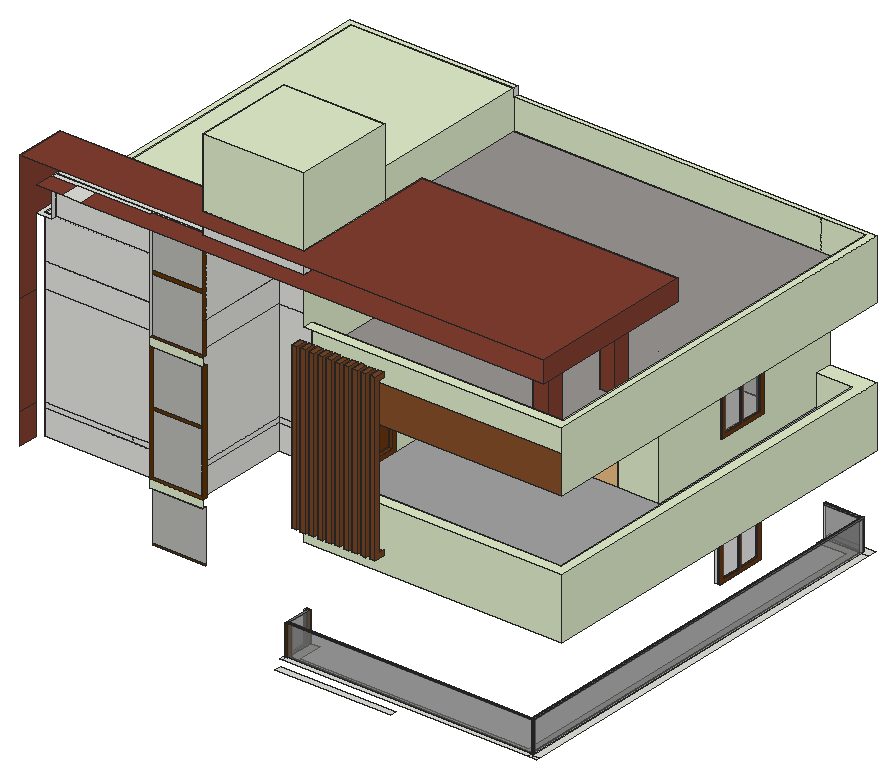
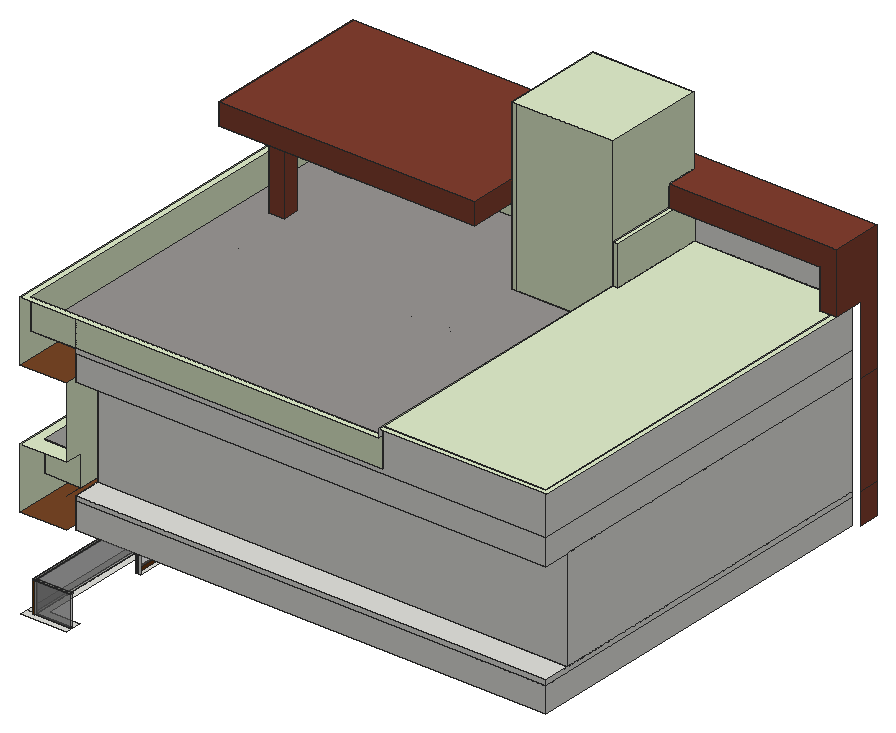
# SketchUp Ruby script. Lengths in inches.
U = 1.inch
M = Sketchup.active_model
def pt(a) = Geom::Point3d.new(a.map { |v| v * U })
def face(e, loops, mat)
  f = e.add_face(loops[0].map { |a| pt(a) })
  loops[1..].each { |l| e.add_face(l.map { |a| pt(a) }).erase! }
  f.material = f.back_material = mat if mat
  f
end
# faces: each face lists its corners as indices into pts; further lists are holes
def faces(e, pts, list, mat = nil) = list.each { |f| face(e, (f[0].is_a?(Array) ? f : [f]).map { |l| l.map { |i| pts[i] } }, mat) }
# xy, xz, yz: faces in a plane at the given z, y or x. An outline is a flat list of corners, or four numbers for a rectangle; further outlines are holes
def ring(l) = l.size == 4 ? [[l[0], l[1]], [l[2], l[1]], [l[2], l[3]], [l[0], l[3]]] : l.each_slice(2).to_a
def flat(e, list, mat, &to3) = list.each { |f| face(e, (f[0].is_a?(Array) ? f : [f]).map { |l| ring(l).map { |u, v| to3.(u, v) } }, mat) }
def xy(e, z, list, mat = nil) = flat(e, list, mat) { |x, y| [x, y, z] }
def xz(e, y, list, mat = nil) = flat(e, list, mat) { |x, z| [x, y, z] }
def yz(e, x, list, mat = nil) = flat(e, list, mat) { |y, z| [x, y, z] }
def lines(e, pts, list) = list.each { |a, b| e.add_line(pt(pts[a]), pt(pts[b])) }
# prism: a flat outline (further loops are holes) pulled along v
def prism(e, loops, v, mat = nil)
  f = face(e, loops, mat); d = Geom::Vector3d.new(v.map { |x| x * U })
  f.pushpull(f.normal.samedirection?(d) ? d.length : -d.length)
end
def box(e, o, s, mat = nil) = prism(e, [[o, [o[0] + s[0], o[1], o[2]], [o[0] + s[0], o[1] + s[1], o[2]], [o[0], o[1] + s[1], o[2]]]], [0, 0, s[2]], mat)
def at(x, y, z, deg = 0) = Geom::Transformation.translation(pt([x, y, z])) * Geom::Transformation.rotation(ORIGIN, Z_AXIS, deg.degrees)
def axes(o, x, y, z) = Geom::Transformation.new([*x, 0, *y, 0, *z, 0, *pt(o).to_a, 1])
def part(name) = M.definitions.add(name)
# library, detail: a bought-in or finely detailed component or shape, given as its bounding box
def library(name, o, s) = part(name).tap { |d| box(d.entities, o, s) }
def detail(e, o, s) = box(e.add_group.entities, o, s)
def put(e, d, t, mat = nil) = e.add_instance(d, t).tap { |i| i.material = mat if mat }
def group(e, t, mat = nil) = e.add_group.tap { |g| g.transformation = t; g.material = mat if mat }.entities
root = M.entities
M.materials.add("[Color A08]").color = [102, 52, 0]
M.materials.add("[Color C08]").color = [82, 45, 0]
M.materials.add("[Concrete Aggregate Smoke]").color = [154, 150, 148]
M.materials.add("[Metal Seamed]").color = [118, 119, 115]
M.materials.add("[Mirror 01]").color = [185, 185, 181]
M.materials.add("[Stone Vein Gray]").color = [166, 165, 165]
M.materials.add("[Translucent Glass Gray]").color = [128, 128, 128]
M.materials["[Translucent Glass Gray]"].alpha = 0.5
M.materials.add("[Wood Board Cork]").color = [130, 63, 47]
M.materials.add("[Wood Lumber ButtJoined]").color = [225, 238, 204]
M.materials.add("[Wood Veneer 01]1").color = [120, 70, 37]
M.materials.add("[Wood Veneer 02]").color = [107, 55, 17]
c1 = part("Group\#4")
xy(c1.entities,0,[[0,0,21.9375,1.125]],"[Wood Veneer 02]")
xy(c1.entities,1.52,[[1.52,0,10.45,1.125],[10.97,0,20.42,1.125]],"[Wood Veneer 02]")
xy(c1.entities,22.11,[[1.52,0,10.45,1.125],[10.97,0,20.42,1.125]],"[Wood Veneer 02]")
xy(c1.entities,23.625,[[0,0,21.9375,1.125]],"[Wood Veneer 02]")
xz(c1.entities,0,[[[0,0,21.9375,23.625],[10.97,1.52,20.42,22.11],[1.52,1.52,10.45,22.11]]],"[Wood Veneer 02]")
xz(c1.entities,1.125,[[1.52,1.52,10.45,22.11],[10.97,1.52,20.42,22.11]],"[Translucent Glass Gray]")
xz(c1.entities,1.125,[[[0,0,21.9375,23.625],[10.97,1.52,20.42,22.11],[1.52,1.52,10.45,22.11]]],"[Wood Veneer 02]")
yz(c1.entities,0,[[0,0,1.125,23.625]],"[Wood Veneer 02]")
yz(c1.entities,1.52,[[0,1.52,1.125,22.11]],"[Wood Veneer 02]")
yz(c1.entities,10.45,[[0,1.52,1.125,22.11]],"[Wood Veneer 02]")
yz(c1.entities,10.97,[[0,1.52,1.125,22.11]],"[Wood Veneer 02]")
yz(c1.entities,20.42,[[0,1.52,1.125,22.11]],"[Wood Veneer 02]")
yz(c1.entities,21.9375,[[0,0,1.125,23.625]],"[Wood Veneer 02]")
c2 = part("Group\#2")
xy(c2.entities,0,[[0,0,48,3.1875]],"[Wood Veneer 02]")
xy(c2.entities,5.53,[[5.53,0,42.47,3.1875]],"[Wood Veneer 02]")
xy(c2.entities,78.47,[[5.53,0,42.47,3.1875]],"[Wood Veneer 02]")
xy(c2.entities,84,[[0,0,48,3.1875]],"[Wood Veneer 02]")
xz(c2.entities,0,[[[0,0,48,84],[5.53,5.53,42.47,78.47]]],"[Wood Veneer 02]")
xz(c2.entities,3.1875,[[[0,0,48,84],[5.53,5.53,42.47,78.47]],[5.53,5.53,42.47,78.47]],"[Wood Veneer 02]")
yz(c2.entities,0,[[0,0,3.1875,84]],"[Wood Veneer 02]")
yz(c2.entities,5.53,[[0,5.53,3.1875,78.47]],"[Wood Veneer 02]")
yz(c2.entities,42.47,[[0,5.53,3.1875,78.47]],"[Wood Veneer 02]")
yz(c2.entities,48,[[0,0,3.1875,84]],"[Wood Veneer 02]")
c3 = library("Group\#5",[0,0,0],[60,3.4375,84])
xy(root,173.23,[[371.79,122.6875,508.29,131.0625]])
xy(root,181.0625,[[370.4375,131.0625,370.4375,168.5625,372.75,168.5625,372.75,136.5625,373.625,136.5625,373.625,131.0625],[373.625,131.0625,664.26,136.5625],[664.26,131.0625,664.26,136.5625,667.0625,136.5625,667.0625,134.5625,675.3125,134.5625,675.3125,131.0625],[667.0625,134.5625,675.3125,622.04],[372.75,136.5625,372.75,168.5625,370.4375,168.5625,370.4375,170.75,375.22,170.75,375.22,139.125,378.16,139.125,664.26,137.39,664.26,136.5625],
  [664.26,136.5625,667.0625,624.5625],[664.26,137.39,664.26,622.04,621.4375,622.04,621.4375,612.27,656.91,612.27,656.91,142.1875,385.875,142.1875,385.875,170.75,375.22,170.75,375.22,139.125,378.16,139.125],[667.0625,622.04,675.3125,622.04,675.3125,631.8125,621.4375,631.8125,621.4375,624.5625,667.0625,624.5625]])
xy(root,198.99,[[615.4375,469.14,621.4375,529.14]])
xy(root,217.0625,[[372.75,136.5625,375.22,139.125]],"[Color C08]")
xy(root,217.0625,[[375.22,136.5625,375.22,139.125,378.16,139.125,664.26,137.39,664.26,136.5625],[664.26,137.39,667.0625,624.5625],[372.75,139.125,375.22,139.125,375.22,170.75,370.4375,170.75,370.4375,168.5625,372.75,168.5625],[621.4375,622.04,664.26,624.5625]],"[Metal Seamed]")
xy(root,218.3125,[[375.22,136.5625,664.26,136.5625,664.26,137.39,378.16,139.125,375.22,139.125],[664.26,136.5625,667.0625,137.39],[664.26,137.39,667.0625,624.5625],[621.4375,622.04,664.26,624.5625]],"[Metal Seamed]")
xy(root,253.0625,[[364.4375,253.7,370.4375,301.7],[512.99,378.5,572.99,384.5]])
xy(root,258.99,[[615.4375,469.14,621.4375,529.14]])
xy(root,282.65,[[187.94,166.9375,251.25,171.5625]],"[Color A08]")
xy(root,289.0625,[[370.4375,166.9375,621.4375,378.5],[621.4375,166.9375,675.875,631.8125]],"[Wood Veneer 01]1")
xy(root,291.97,[[187.94,166.9375,251.25,171.75]],"[Color A08]")
xy(root,307.4375,[[365.79,154.25,372.22,166.9375],[376.04,154.25,382.47,166.9375],[386.29,154.25,392.72,166.9375],[396.54,154.25,402.97,166.9375],[406.79,154.25,413.22,166.9375],
  [417.04,154.25,423.47,166.9375],[427.29,154.25,433.72,166.9375],[437.54,154.25,443.97,166.9375],[447.79,154.25,454.22,166.9375],[458.04,154.25,464.47,167.53]],"[Wood Veneer 01]1")
xy(root,313.15,[[365.79,160.59,372.22,166.9375],[376.04,160.59,382.47,166.9375],[386.29,160.59,392.72,166.9375],[396.54,160.59,402.97,166.9375],[406.79,160.59,413.22,166.9375],
  [417.04,160.59,423.47,166.9375],[427.29,160.59,433.72,166.9375],[437.54,160.59,443.97,166.9375],[447.79,160.59,454.22,166.9375],[458.04,160.59,464.47,167.53]],"[Wood Veneer 01]1")
xy(root,319.0625,[[59.1875,172.9375,59.1875,625.8125,615.4375,625.8125,615.4375,384.5,364.4375,384.5,364.4375,286.0625,245.25,286.0625,245.25,172.9375]])
xy(root,325.0625,[[59.1875,172.9375,245.25,172.9375,245.25,286.0625,364.4375,286.0625,364.4375,384.5,615.4375,384.5,615.4375,593.4375,59.1875,593.4375],[59.1875,593.4375,615.4375,625.8125]])
xy(root,325.0625,[[370.4375,180.44,663.99,180.44,663.99,611.05,621.4375,611.05,621.4375,378.5,572.99,378.5,572.99,384.5,513.3,384.5,513.3,378.5,370.4375,378.5,370.4375,303.3,365.125,303.3,365.125,255.3,370.4375,255.3]],"[Stone Vein Gray]")
xy(root,353.87,[[615.4375,470.21,621.4375,530.21]])
xy(root,361.0625,[[370.4375,166.9375,675.875,166.9375,675.875,631.8125,621.4375,631.8125,621.4375,611.05,663.99,611.05,663.99,180.44,370.4375,180.44]],"[Wood Lumber ButtJoined]")
xy(root,409.0625,[[365.125,255.3,370.4375,303.3],[513.3,378.5,572.99,384.5]])
xy(root,413.87,[[615.4375,470.21,621.4375,530.21]])
xy(root,432.81,[[187.94,166.9375,251.25,171.75]],"[Color A08]")
xy(root,442.28,[[187.94,166.9375,251.25,170.6875]],"[Color A08]")
xy(root,445.0625,[[59.1875,593.4375,615.4375,625.8125]])
xy(root,445.0625,[[370.4375,166.9375,675.875,378.5],[621.4375,378.5,675.875,631.8125]],"[Wood Veneer 01]1")
xy(root,475.0625,[[59.1875,172.9375,59.1875,625.8125,615.4375,625.8125,615.4375,384.5,364.4375,384.5,364.4375,286.0625,245.25,286.0625,245.25,172.9375]])
xy(root,481.0625,[[617.24,197.4,635.87,216.4],[617.24,295.65,635.87,314.27]])
xy(root,481.0625,[[[370.4375,179,667.67,179,667.67,625.8125,251.25,625.8125,251.25,286.0625,370.4375,286.0625],[617.24,197.4,635.87,216.4],[617.24,295.65,635.87,314.27]]],"[Concrete Aggregate Smoke]")
xy(root,495.42,[[365.79,160.59,372.22,166.9375],[376.04,160.59,382.47,166.9375],[386.29,160.59,392.72,166.9375],[396.54,160.59,402.97,166.9375],[406.79,160.59,413.22,166.9375],
  [417.04,160.59,423.47,166.9375],[427.29,160.59,433.72,166.9375],[437.54,160.59,443.97,166.9375],[447.79,160.59,454.22,166.9375],[458.04,160.59,464.47,166.9375]],"[Wood Veneer 01]1")
xy(root,501.86,[[365.79,154.25,372.22,166.9375],[376.04,154.25,382.47,166.9375],[386.29,154.25,392.72,166.9375],[396.54,154.25,402.97,166.9375],[406.79,154.25,413.22,166.9375],
  [417.04,154.25,423.47,166.9375],[427.29,154.25,433.72,166.9375],[437.54,154.25,443.97,166.9375],[447.79,154.25,454.22,166.9375],[458.04,154.25,464.47,166.9375]],"[Wood Veneer 01]1")
xy(root,517.0625,[[370.4375,166.9375,675.875,166.9375,675.875,631.8125,251.25,631.8125,251.25,625.8125,667.67,625.8125,667.67,179,370.4375,179]],"[Wood Lumber ButtJoined]")
xy(root,526.5,[[53.1875,166.9375,53.1875,203.125,59.1875,203.125,59.1875,172.9375,72.33,172.9375,72.33,166.9375],[59.1875,172.9375,72.33,203.125]])
xy(root,526.5,[[72.33,172.9375,245.25,172.9375,245.25,286.0625,251.25,286.0625,251.25,625.8125,59.1875,625.8125,59.1875,203.125,72.33,203.125],[53.1875,203.125,59.1875,203.125,59.1875,625.8125,251.25,625.8125,251.25,631.8125,53.1875,631.8125]],"[Wood Lumber ButtJoined]")
xy(root,572.45,[[103.04,144.0625,124.63,166.9375],[72.33,166.9375,72.33,172.9375,245.25,172.9375,245.25,203.125,251.25,203.125,251.25,170.6875,187.94,170.6875,187.94,166.9375],[72.33,172.9375,245.25,203.125]])
xy(root,572.45,[[72.33,144.0625,103.04,166.9375],[124.63,144.0625,124.63,166.9375,187.94,166.9375,187.94,170.6875,251.25,170.6875,251.25,166.9375,370.4375,166.9375,370.4375,341.9375,672.375,341.9375,672.375,144.0625]],"[Wood Board Cork]")
xy(root,572.45,[[245.25,203.125,251.25,286.0625]],"[Wood Lumber ButtJoined]")
xy(root,572.6875,[[617.24,295.65,635.87,314.27]])
xy(root,578.8125,[[617.24,197.4,635.87,216.4]])
xy(root,597.6875,[[53.1875,144.0625,672.375,144.0625,672.375,341.9375,370.4375,341.9375,370.4375,166.9375,251.25,166.9375,251.25,203.125,53.1875,203.125]],"[Wood Board Cork]")
xy(root,679.6875,[[251.25,166.9375,370.4375,286.0625]],"[Wood Lumber ButtJoined]")
xz(root,136.5625,[[372.75,181.0625,375.22,217.0625],[664.26,181.0625,667.0625,218.3125]],"[Color C08]")
xz(root,136.5625,[[375.22,217.0625,664.26,218.3125]],"[Metal Seamed]")
xz(root,136.5625,[[375.22,181.0625,664.26,217.0625]],"[Translucent Glass Gray]")
xz(root,137.39,[[664.26,217.0625,667.0625,218.3125]],"[Metal Seamed]")
xz(root,139.125,[[375.22,181.0625,378.16,217.0625]],"[Color A08]")
xz(root,139.125,[[375.22,217.0625,378.16,218.3125]],"[Metal Seamed]")
xz(root,154.25,[[365.79,307.4375,372.22,501.86],[376.04,307.4375,382.47,501.86],[386.29,307.4375,392.72,501.86],[396.54,307.4375,402.97,501.86],[406.79,307.4375,413.22,501.86],
  [417.04,307.4375,423.47,501.86],[427.29,307.4375,433.72,501.86],[437.54,307.4375,443.97,501.86],[447.79,307.4375,454.22,501.86],[458.04,307.4375,464.47,501.86]],"[Wood Veneer 01]1")
xz(root,160.59,[[365.79,313.15,372.22,495.42],[376.04,313.15,382.47,495.42],[386.29,313.15,392.72,495.42],[396.54,313.15,402.97,495.42],[406.79,313.15,413.22,495.42],
  [417.04,313.15,423.47,495.42],[427.29,313.15,433.72,495.42],[437.54,313.15,443.97,495.42],[447.79,313.15,454.22,495.42],[458.04,313.15,464.47,495.42]],"[Wood Veneer 01]1")
xz(root,166.9375,[[365.79,307.4375,370.4375,313.15],[370.4375,307.4375,372.22,313.15],[251.25,572.45,370.4375,597.6875]])
xz(root,166.9375,[[187.94,282.65,251.25,291.97],[[370.4375,289.0625,675.875,289.0625,675.875,361.0625,370.4375,361.0625,370.4375,313.15,372.22,313.15,372.22,307.4375,370.4375,307.4375],[376.04,307.4375,382.47,313.15],[386.29,307.4375,392.72,313.15],[396.54,307.4375,402.97,313.15],[406.79,307.4375,413.22,313.15],[417.04,307.4375,423.47,313.15],[427.29,307.4375,433.72,313.15],[437.54,307.4375,443.97,313.15],[447.79,307.4375,454.22,313.15]],[187.94,432.81,251.25,442.28],[251.25,597.6875,370.4375,679.6875]],"[Wood Lumber ButtJoined]")
xz(root,167.53,[[458.04,307.4375,464.47,313.15]])
xz(root,168.5625,[[370.4375,181.0625,372.75,217.0625]],"[Color A08]")
xz(root,170.6875,[[187.94,507.37,251.25,511.61]],"[Color A08]")
xz(root,170.6875,[[187.94,442.28,251.25,507.37],[187.94,511.61,251.25,572.45]],"[Mirror 01]")
xz(root,170.75,[[370.4375,181.0625,375.22,217.0625]],"[Color A08]")
xz(root,171.5625,[[187.94,219.24,251.25,222.23]],"[Color A08]")
xz(root,171.5625,[[187.94,222.23,251.25,282.65]],"[Mirror 01]")
xz(root,171.75,[[187.94,362.39,251.25,365.47]],"[Color A08]")
xz(root,171.75,[[187.94,291.97,251.25,362.39],[187.94,365.47,251.25,432.81]],"[Mirror 01]")
xz(root,172.9375,[[59.1875,289.0625,245.25,319.0625],[59.1875,319.0625,163.16,325.0625],[163.16,319.0625,186.28,325.0625],[186.28,319.0625,245.25,325.0625],[59.1875,325.0625,245.25,445.0625],
  [59.1875,445.0625,245.25,475.0625],[59.1875,475.0625,245.25,526.5],[72.33,526.5,245.25,572.45]])
xz(root,179,[[370.4375,481.0625,667.67,517.0625]],"[Wood Lumber ButtJoined]")
xz(root,180.44,[[370.4375,325.0625,663.99,361.0625]])
xz(root,197.4,[[617.24,481.0625,635.87,578.8125]],"[Wood Board Cork]")
xz(root,203.125,[[53.1875,526.5,53.1875,597.6875,251.25,597.6875,251.25,572.45,72.33,572.45,72.33,526.5]],"[Wood Board Cork]")
xz(root,216.4,[[617.24,481.0625,635.87,578.8125]],"[Wood Board Cork]")
xz(root,255.3,[[365.125,325.0625,370.4375,409.0625]])
xz(root,286.0625,[[245.25,289.0625,364.4375,319.0625],[245.25,319.0625,364.4375,325.0625],[245.25,325.0625,364.4375,445.0625],[245.25,445.0625,364.4375,475.0625],[245.25,475.0625,245.25,526.5,251.25,526.5,251.25,481.0625,364.4375,481.0625,364.4375,475.0625]])
xz(root,286.0625,[[251.25,481.0625,364.4375,679.6875],[364.4375,481.0625,370.4375,679.6875],[245.25,526.5,251.25,572.45]],"[Wood Lumber ButtJoined]")
xz(root,295.65,[[617.24,481.0625,635.87,572.6875]],"[Wood Board Cork]")
xz(root,303.3,[[365.125,325.0625,370.4375,409.0625]])
xz(root,314.27,[[617.24,481.0625,635.87,572.6875]],"[Wood Board Cork]")
xz(root,341.9375,[[370.4375,572.45,672.375,597.6875]],"[Wood Board Cork]")
xz(root,378.5,[[370.4375,325.0625,513.3,325.0625,513.3,409.0625,572.99,409.0625,572.99,325.0625,621.4375,325.0625,621.4375,445.0625,370.4375,445.0625]],"[Wood Lumber ButtJoined]")
xz(root,384.5,[[364.4375,289.0625,615.4375,319.0625],[364.4375,319.0625,615.4375,325.0625],[364.4375,325.0625,364.4375,445.0625,615.4375,445.0625,615.4375,325.0625,572.99,325.0625,572.99,409.0625,513.3,409.0625,513.3,325.0625],[364.4375,445.0625,615.4375,475.0625]])
xz(root,469.14,[[615.4375,198.99,621.4375,258.99]])
xz(root,470.21,[[615.4375,353.87,621.4375,413.87]])
xz(root,529.14,[[615.4375,198.99,621.4375,258.99]])
xz(root,530.21,[[615.4375,353.87,621.4375,413.87]])
xz(root,593.4375,[[59.1875,325.0625,615.4375,445.0625]])
xz(root,611.05,[[621.4375,325.0625,663.99,361.0625]],"[Wood Lumber ButtJoined]")
xz(root,622.04,[[621.4375,217.0625,664.26,218.3125]],"[Metal Seamed]")
xz(root,622.04,[[621.4375,181.0625,664.26,217.0625]],"[Translucent Glass Gray]")
xz(root,624.5625,[[664.26,181.0625,667.0625,217.0625]],"[Color A08]")
xz(root,624.5625,[[621.4375,217.0625,664.26,218.3125],[664.26,217.0625,667.0625,218.3125]],"[Metal Seamed]")
xz(root,624.5625,[[621.4375,181.0625,664.26,217.0625]],"[Translucent Glass Gray]")
xz(root,625.8125,[[59.1875,289.0625,615.4375,319.0625],[59.1875,319.0625,615.4375,325.0625],[59.1875,445.0625,615.4375,475.0625],[59.1875,475.0625,615.4375,475.0625,615.4375,481.0625,251.25,481.0625,251.25,526.5,59.1875,526.5]])
xz(root,625.8125,[[251.25,481.0625,615.4375,517.0625],[615.4375,481.0625,667.67,517.0625]],"[Wood Lumber ButtJoined]")
yz(root,53.1875,[[144.0625,289.0625,166.9375,325.0625],[144.0625,325.0625,166.9375,445.0625],[144.0625,445.0625,144.0625,597.6875,203.125,597.6875,203.125,526.5,166.9375,526.5,166.9375,445.0625]],"[Wood Board Cork]")
yz(root,59.1875,[[172.9375,289.0625,625.8125,319.0625],[172.9375,319.0625,625.8125,325.0625],[172.9375,325.0625,593.4375,445.0625],[172.9375,445.0625,625.8125,475.0625],[172.9375,475.0625,625.8125,526.5]])
yz(root,72.33,[[166.9375,526.5,172.9375,572.45],[172.9375,526.5,203.125,572.45]])
yz(root,187.94,[[166.9375,442.28,170.6875,572.45]])
yz(root,187.94,[[166.9375,291.97,171.75,432.81]],"[Color A08]")
yz(root,245.25,[[172.9375,289.0625,286.0625,319.0625],[172.9375,319.0625,286.0625,325.0625],[172.9375,325.0625,286.0625,445.0625],[172.9375,445.0625,286.0625,475.0625],[172.9375,475.0625,286.0625,526.5]])
yz(root,245.25,[[172.9375,526.5,286.0625,572.45]],"[Wood Lumber ButtJoined]")
yz(root,251.25,[[170.6875,481.0625,286.0625,572.45],[625.8125,517.0625,631.8125,526.5],[166.9375,572.45,203.125,597.6875]])
yz(root,251.25,[[166.9375,291.97,171.75,432.81],[166.9375,442.28,170.6875,481.0625],[166.9375,481.0625,170.6875,572.45]],"[Color A08]")
yz(root,251.25,[[286.0625,481.0625,625.8125,526.5],[203.125,572.45,203.125,597.6875,166.9375,597.6875,166.9375,679.6875,286.0625,679.6875,286.0625,572.45]],"[Wood Lumber ButtJoined]")
yz(root,364.4375,[[286.0625,289.0625,384.5,319.0625],[286.0625,319.0625,384.5,325.0625],[286.0625,325.0625,384.5,445.0625],[286.0625,445.0625,384.5,475.0625]])
yz(root,365.125,[[255.3,325.0625,303.3,409.0625]])
yz(root,365.79,[[154.25,307.4375,154.25,501.86,166.9375,501.86,166.9375,495.42,160.59,495.42,160.59,313.15,166.9375,313.15,166.9375,307.4375]],"[Wood Veneer 01]1")
yz(root,370.4375,[[166.9375,181.0625,168.5625,217.0625],[168.5625,181.0625,170.75,217.0625],[166.9375,325.0625,180.44,361.0625],[166.9375,572.45,286.0625,597.6875]])
yz(root,370.4375,[[286.0625,572.45,341.9375,597.6875]],"[Wood Board Cork]")
yz(root,370.4375,[[180.44,325.0625,255.3,325.0625,255.3,409.0625,303.3,409.0625,303.3,325.0625,378.5,325.0625,378.5,445.0625,166.9375,445.0625,166.9375,361.0625,180.44,361.0625],[179,481.0625,286.0625,481.0625,286.0625,572.45,166.9375,572.45,166.9375,517.0625,179,517.0625],[166.9375,597.6875,286.0625,679.6875]],"[Wood Lumber ButtJoined]")
yz(root,372.22,[[154.25,307.4375,166.9375,307.4375,166.9375,313.15,160.59,313.15,160.59,495.42,166.9375,495.42,166.9375,501.86,154.25,501.86]],"[Wood Veneer 01]1")
yz(root,372.75,[[136.5625,181.0625,139.125,217.0625]],"[Color C08]")
yz(root,372.75,[[139.125,181.0625,168.5625,217.0625]],"[Translucent Glass Gray]")
yz(root,375.22,[[136.5625,217.0625,139.125,218.3125]],"[Metal Seamed]")
yz(root,375.22,[[139.125,181.0625,170.75,217.0625]],"[Translucent Glass Gray]")
yz(root,376.04,[[154.25,307.4375,154.25,501.86,166.9375,501.86,166.9375,495.42,160.59,495.42,160.59,313.15,166.9375,313.15,166.9375,307.4375]],"[Wood Veneer 01]1")
yz(root,382.47,[[154.25,307.4375,166.9375,307.4375,166.9375,313.15,160.59,313.15,160.59,495.42,166.9375,495.42,166.9375,501.86,154.25,501.86]],"[Wood Veneer 01]1")
yz(root,386.29,[[154.25,307.4375,154.25,501.86,166.9375,501.86,166.9375,495.42,160.59,495.42,160.59,313.15,166.9375,313.15,166.9375,307.4375]],"[Wood Veneer 01]1")
yz(root,392.72,[[154.25,307.4375,166.9375,307.4375,166.9375,313.15,160.59,313.15,160.59,495.42,166.9375,495.42,166.9375,501.86,154.25,501.86]],"[Wood Veneer 01]1")
yz(root,396.54,[[154.25,307.4375,154.25,501.86,166.9375,501.86,166.9375,495.42,160.59,495.42,160.59,313.15,166.9375,313.15,166.9375,307.4375]],"[Wood Veneer 01]1")
yz(root,402.97,[[154.25,307.4375,166.9375,307.4375,166.9375,313.15,160.59,313.15,160.59,495.42,166.9375,495.42,166.9375,501.86,154.25,501.86]],"[Wood Veneer 01]1")
yz(root,406.79,[[154.25,307.4375,154.25,501.86,166.9375,501.86,166.9375,495.42,160.59,495.42,160.59,313.15,166.9375,313.15,166.9375,307.4375]],"[Wood Veneer 01]1")
yz(root,413.22,[[154.25,307.4375,166.9375,307.4375,166.9375,313.15,160.59,313.15,160.59,495.42,166.9375,495.42,166.9375,501.86,154.25,501.86]],"[Wood Veneer 01]1")
yz(root,417.04,[[154.25,307.4375,154.25,501.86,166.9375,501.86,166.9375,495.42,160.59,495.42,160.59,313.15,166.9375,313.15,166.9375,307.4375]],"[Wood Veneer 01]1")
yz(root,423.47,[[154.25,307.4375,166.9375,307.4375,166.9375,313.15,160.59,313.15,160.59,495.42,166.9375,495.42,166.9375,501.86,154.25,501.86]],"[Wood Veneer 01]1")
yz(root,427.29,[[154.25,307.4375,154.25,501.86,166.9375,501.86,166.9375,495.42,160.59,495.42,160.59,313.15,166.9375,313.15,166.9375,307.4375]],"[Wood Veneer 01]1")
yz(root,433.72,[[154.25,307.4375,166.9375,307.4375,166.9375,313.15,160.59,313.15,160.59,495.42,166.9375,495.42,166.9375,501.86,154.25,501.86]],"[Wood Veneer 01]1")
yz(root,437.54,[[154.25,307.4375,154.25,501.86,166.9375,501.86,166.9375,495.42,160.59,495.42,160.59,313.15,166.9375,313.15,166.9375,307.4375]],"[Wood Veneer 01]1")
yz(root,443.97,[[154.25,307.4375,166.9375,307.4375,166.9375,313.15,160.59,313.15,160.59,495.42,166.9375,495.42,166.9375,501.86,154.25,501.86]],"[Wood Veneer 01]1")
yz(root,447.79,[[154.25,307.4375,154.25,501.86,166.9375,501.86,166.9375,495.42,160.59,495.42,160.59,313.15,166.9375,313.15,166.9375,307.4375]],"[Wood Veneer 01]1")
yz(root,454.22,[[154.25,307.4375,166.9375,307.4375,166.9375,313.15,160.59,313.15,160.59,495.42,166.9375,495.42,166.9375,501.86,154.25,501.86]],"[Wood Veneer 01]1")
yz(root,458.04,[[154.25,307.4375,154.25,501.86,166.9375,501.86,166.9375,495.42,160.59,495.42,160.59,313.15,167.53,313.15,167.53,307.4375]],"[Wood Veneer 01]1")
yz(root,464.47,[[154.25,307.4375,167.53,307.4375,167.53,313.15,160.59,313.15,160.59,495.42,166.9375,495.42,166.9375,501.86,154.25,501.86]],"[Wood Veneer 01]1")
yz(root,513.3,[[378.5,325.0625,384.5,409.0625]])
yz(root,572.99,[[378.5,325.0625,384.5,409.0625]])
yz(root,615.4375,[[384.5,289.0625,625.8125,319.0625],[384.5,319.0625,625.8125,325.0625],[[384.5,325.0625,593.4375,445.0625],[470.21,353.87,530.21,413.87]],[384.5,445.0625,625.8125,475.0625]])
yz(root,617.24,[[197.4,481.0625,216.4,578.8125],[295.65,481.0625,314.27,572.6875]],"[Wood Board Cork]")
yz(root,621.4375,[[622.04,217.0625,624.5625,218.3125]],"[Metal Seamed]")
yz(root,621.4375,[[[378.5,325.0625,611.05,325.0625,611.05,361.0625,631.8125,361.0625,631.8125,445.0625,378.5,445.0625],[470.21,353.87,530.21,413.87]]],"[Wood Lumber ButtJoined]")
yz(root,635.87,[[197.4,481.0625,216.4,578.8125],[295.65,481.0625,314.27,572.6875]],"[Wood Board Cork]")
yz(root,663.99,[[180.44,325.0625,611.05,361.0625]])
yz(root,664.26,[[136.5625,181.0625,137.39,217.0625],[622.04,181.0625,624.5625,217.0625]])
yz(root,664.26,[[136.5625,217.0625,137.39,218.3125],[137.39,217.0625,622.04,218.3125],[622.04,217.0625,624.5625,218.3125]],"[Metal Seamed]")
yz(root,664.26,[[137.39,181.0625,622.04,217.0625]],"[Translucent Glass Gray]")
yz(root,667.0625,[[136.5625,181.0625,137.39,218.3125]],"[Color C08]")
yz(root,667.0625,[[137.39,217.0625,624.5625,218.3125]],"[Metal Seamed]")
yz(root,667.0625,[[137.39,181.0625,624.5625,217.0625]],"[Translucent Glass Gray]")
yz(root,667.67,[[179,481.0625,625.8125,517.0625]],"[Wood Lumber ButtJoined]")
yz(root,672.375,[[144.0625,572.45,341.9375,597.6875]],"[Wood Board Cork]")
yz(root,675.875,[[166.9375,289.0625,631.8125,361.0625],[166.9375,445.0625,631.8125,517.0625]],"[Wood Lumber ButtJoined]")
p = [[664.26,137.39,181.0625],[378.16,139.125,181.0625],[378.16,139.125,217.0625],[664.26,137.39,217.0625],[378.16,139.125,218.3125],[664.26,137.39,218.3125],
  [621.4375,631.8125,325.0625],[621.4375,611.05,325.0625],[370.4375,378.5,445.0625],[370.4375,378.5,481.0625],[411.54,384.5,481.0625],[411.54,384.5,475.0625],
  [615.4375,384.5,475.0625],[615.4375,384.5,481.0625],[364.4375,384.5,475.0625],[364.4375,384.5,481.0625]]
faces(root,p,[[0,1,2,3]],"[Translucent Glass Gray]")
faces(root,p,[[3,2,4,5]],"[Metal Seamed]")
lines(root,p,[[6,7],[8,9],[10,11],[12,13],[14,15]])
put(root,c1,axes([621.4375,468.59,198.99],[0,2.76,0],[-1.84,0,0],[0,0,2.53968]))
put(root,c2,axes([370.4375,255.64,325.0625],[0,0.99284,0],[-1.31328,0,0],[0,0,1.00224]))
put(root,c3,at(512.99,378.5,325.0625))
put(root,c1,axes([623.51,469.66,353.87],[0,2.76,0],[-1.84,0,0],[0,0,2.53968]))
